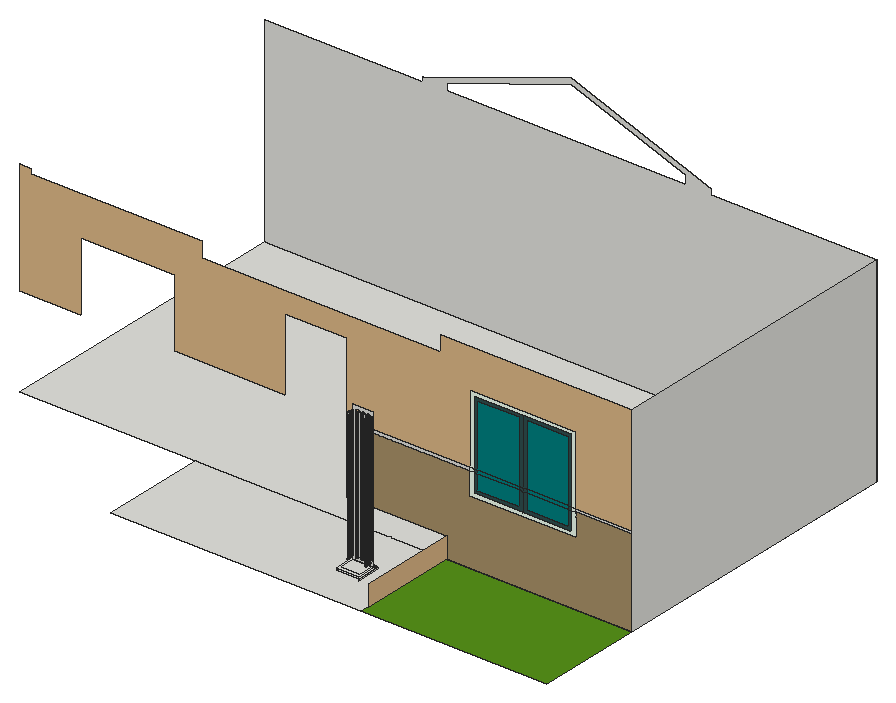
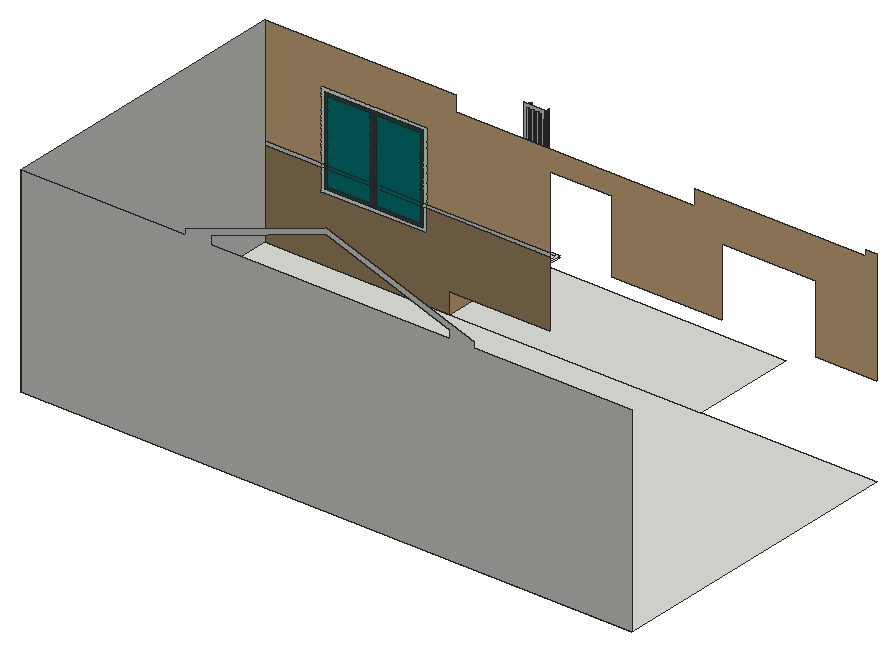
# SketchUp Ruby script. Lengths in inches.
U = 1.inch
M = Sketchup.active_model
def pt(a) = Geom::Point3d.new(a.map { |v| v * U })
def face(e, loops, mat)
  f = e.add_face(loops[0].map { |a| pt(a) })
  loops[1..].each { |l| e.add_face(l.map { |a| pt(a) }).erase! }
  f.material = f.back_material = mat if mat
  f
end
# faces: each face lists its corners as indices into pts; further lists are holes
def faces(e, pts, list, mat = nil) = list.each { |f| face(e, (f[0].is_a?(Array) ? f : [f]).map { |l| l.map { |i| pts[i] } }, mat) }
# xy, xz, yz: faces in a plane at the given z, y or x. An outline is a flat list of corners, or four numbers for a rectangle; further outlines are holes
def ring(l) = l.size == 4 ? [[l[0], l[1]], [l[2], l[1]], [l[2], l[3]], [l[0], l[3]]] : l.each_slice(2).to_a
def flat(e, list, mat, &to3) = list.each { |f| face(e, (f[0].is_a?(Array) ? f : [f]).map { |l| ring(l).map { |u, v| to3.(u, v) } }, mat) }
def xy(e, z, list, mat = nil) = flat(e, list, mat) { |x, y| [x, y, z] }
def xz(e, y, list, mat = nil) = flat(e, list, mat) { |x, z| [x, y, z] }
def yz(e, x, list, mat = nil) = flat(e, list, mat) { |y, z| [x, y, z] }
def lines(e, pts, list) = list.each { |a, b| e.add_line(pt(pts[a]), pt(pts[b])) }
# prism: a flat outline (further loops are holes) pulled along v
def prism(e, loops, v, mat = nil)
  f = face(e, loops, mat); d = Geom::Vector3d.new(v.map { |x| x * U })
  f.pushpull(f.normal.samedirection?(d) ? d.length : -d.length)
end
def box(e, o, s, mat = nil) = prism(e, [[o, [o[0] + s[0], o[1], o[2]], [o[0] + s[0], o[1] + s[1], o[2]], [o[0], o[1] + s[1], o[2]]]], [0, 0, s[2]], mat)
def at(x, y, z, deg = 0) = Geom::Transformation.translation(pt([x, y, z])) * Geom::Transformation.rotation(ORIGIN, Z_AXIS, deg.degrees)
def axes(o, x, y, z) = Geom::Transformation.new([*x, 0, *y, 0, *z, 0, *pt(o).to_a, 1])
def part(name) = M.definitions.add(name)
# library, detail: a bought-in or finely detailed component or shape, given as its bounding box
def library(name, o, s) = part(name).tap { |d| box(d.entities, o, s) }
def detail(e, o, s) = box(e.add_group.entities, o, s)
def put(e, d, t, mat = nil) = e.add_instance(d, t).tap { |i| i.material = mat if mat }
def group(e, t, mat = nil) = e.add_group.tap { |g| g.transformation = t; g.material = mat if mat }.entities
root = M.entities
M.materials.add("[0036_BurlyWood]").color = [222, 184, 135]
M.materials.add("[0066_Honeydew]").color = [240, 255, 240]
M.materials.add("[0078_DarkSlateGray]").color = [47, 79, 79]
M.materials.add("[0079_Teal]").color = [0, 128, 128]
M.materials.add("[Stone Sandstone Ashlar Light]").color = [168, 145, 104]
M.materials.add("[Vegetation Honey Locust]").color = [86, 145, 25]
xy(root,0,[[103.43,1.91,251.04,64.75],[0,64.75,360,244.75]])
xy(root,0,[[251.04,1.91,360,64.75]],"[Vegetation Honey Locust]")
xy(root,12.13,[[231.46,8.1,244.45,21.09]])
xy(root,13.17,[[[231.46,8.1,244.45,21.09],[232.25,9.67,243.67,19.51]]])
xz(root,19.51,[[[232.25,13.17,243.67,94.95],[240.91,14.97,241.17,15,241.4,15.09,241.61,15.24,241.76,15.42,241.86,15.64,241.9,15.875,241.9,92.25,241.86,92.48,241.76,92.7,241.61,92.89,241.4,93.03,241.17,93.12,240.91,93.15,240.66,93.12,240.42,93.03,240.22,92.89,240.06,92.7,239.96,92.48,239.93,92.25,239.93,15.875,239.96,15.64,240.06,15.42,240.22,15.24,240.42,15.09,240.66,15],[235.01,14.97,235.26,15,235.5,15.09,235.7,15.24,235.86,15.42,235.96,15.64,235.99,15.875,235.99,92.25,235.96,92.48,235.86,92.7,235.7,92.89,235.5,93.03,235.26,93.12,235.01,93.15,234.75,93.12,234.51,93.03,234.31,92.89,234.15,92.7,234.05,92.48,234.02,92.25,234.02,15.875,234.05,15.64,234.15,15.42,234.31,15.24,234.51,15.09,234.75,15],[237.96,14.97,238.21,15,238.45,15.09,238.65,15.24,238.8125,15.42,238.91,15.64,238.94,15.875,238.94,92.25,238.91,92.48,238.8125,92.7,238.65,92.89,238.45,93.03,238.21,93.12,237.96,93.15,237.7,93.12,237.47,93.03,237.26,92.89,237.11,92.7,237.01,92.48,236.97,92.25,236.97,15.875,237.01,15.64,237.11,15.42,237.26,15.24,237.47,15.09,237.7,15]]])
xz(root,21.09,[[231.46,12.13,244.45,13.02],[231.46,13.02,244.45,13.17]])
xz(root,21.61,[[230.94,11.46,244.97,12.13]])
xz(root,64.75,[[191.99,51.19,264.92,53.19],[326.96,51.19,360,53.19]])
xz(root,64.75,[[0,53.19,35.4,53.19,35.4,93.75,90.9,93.75,90.9,53.19,155.99,53.19,155.99,96,191.99,96,191.99,53.19,264.92,53.19,264.92,93.75,326.96,93.75,326.96,53.19,360,53.19,360,117,247.8,117,247.8,108.125,106.86,108.125,106.86,117,6.32,117,6.32,120,0,120]],"[0036_BurlyWood]")
xz(root,64.75,[[264.92,38.25,326.96,38.25,326.96,51.19,324.96,51.19,324.96,40.25,266.92,40.25,266.92,51.19,264.92,51.19],[264.92,51.19,266.92,53.19],[324.96,51.19,326.96,53.19],[264.92,53.19,266.92,53.19,266.92,91.75,324.96,91.75,324.96,53.19,326.96,53.19,326.96,93.75,264.92,93.75]],"[0066_Honeydew]")
xz(root,64.75,[[266.92,40.25,295.9375,40.25,295.9375,51.19,293.9375,51.19,293.9375,42.25,268.92,42.25,268.92,51.19,266.92,51.19],[295.9375,40.25,324.96,40.25,324.96,51.19,322.96,51.19,322.96,42.25,297.9375,42.25,297.9375,51.19,295.9375,51.19],[266.92,51.19,268.92,53.19],[293.9375,51.19,295.9375,53.19],[295.9375,51.19,297.9375,53.19],
  [322.96,51.19,324.96,53.19],[266.92,53.19,268.92,53.19,268.92,89.75,293.9375,89.75,293.9375,53.19,295.9375,53.19,295.9375,91.75,266.92,91.75],[295.9375,53.19,297.9375,53.19,297.9375,89.75,322.96,89.75,322.96,53.19,324.96,53.19,324.96,91.75,295.9375,91.75]],"[0078_DarkSlateGray]")
xz(root,64.75,[[268.92,42.25,293.9375,51.19],[297.9375,42.25,322.96,51.19],[268.92,51.19,293.9375,53.19],[297.9375,51.19,322.96,53.19],[268.92,53.19,293.9375,89.75],
  [297.9375,53.19,322.96,89.75]],"[0079_Teal]")
xz(root,64.75,[[251.04,0,360,0,360,51.19,326.96,51.19,326.96,38.25,264.92,38.25,264.92,51.19,191.99,51.19,191.99,12,251.04,12]],"[Stone Sandstone Ashlar Light]")
xz(root,244.75,[[[0,0,0,117,93.16,117,93.16,119.98,93.21,120,180,149.8,262.52,120,262.6,119.97,262.6,117,360,117,360,0],[106.86,117,247.8,117,247.8,122.125,179.96,146.625,106.86,121.52]]])
yz(root,244.97,[[7.58,11.46,21.61,12.13]])
yz(root,251.04,[[7.125,0,64.75,12]],"[0036_BurlyWood]")
yz(root,360,[[64.75,0,244.75,117]])
p = [[231.14,21.41,12.15],[231.2,21.35,12.2],[244.71,21.35,12.2],[244.78,21.41,12.15],[231.11,21.44,12.13],[244.81,21.44,12.13],
  [231.26,21.29,12.27],[244.65,21.29,12.27],[231.32,21.24,12.36],[244.6,21.24,12.36],[231.36,21.1875,12.47],[244.55,21.1875,12.47],
  [231.4,21.15,12.59],[244.52,21.15,12.59],[231.43,21.12,12.73],[244.49,21.12,12.73],[231.45,21.1,12.87],[244.47,21.1,12.87],
  [231.46,21.09,13.02],[244.45,21.09,13.02],[234.88,19.29,15],[234.76,19.09,15.09],[234.88,19.04,15.09],[234.94,19.27,15],
  [235.01,19.02,15.09],[235.01,19.26,15],[235.13,19.04,15.09],[235.07,19.27,15],[235.25,19.09,15.09],[235.13,19.29,15],
  [237.83,19.29,15],[237.71,19.09,15.09],[237.83,19.04,15.09],[237.89,19.27,15],[237.96,19.02,15.09],[237.96,19.26,15],
  [238.09,19.04,15.09],[238.02,19.27,15],[238.2,19.09,15.09],[238.09,19.29,15],[240.78,19.29,15],[240.67,19.09,15.09],
  [240.78,19.04,15.09],[240.85,19.27,15],[240.91,19.02,15.09],[240.91,19.26,15],[241.04,19.04,15.09],[240.98,19.27,15],
  [241.16,19.09,15.09],[241.04,19.29,15],[234.83,19.33,15],[234.66,19.17,15.09],[235.35,19.17,15.09],[235.1875,19.33,15],
  [237.78,19.33,15],[237.61,19.17,15.09],[238.31,19.17,15.09],[238.14,19.33,15],[240.73,19.33,15],[240.5625,19.17,15.09],
  [241.26,19.17,15.09],[241.09,19.33,15],[234.78,19.39,15],[234.58,19.27,15.09],[235.43,19.27,15.09],[235.23,19.39,15],
  [237.74,19.39,15],[237.53,19.27,15.09],[238.38,19.27,15.09],[238.18,19.39,15],[240.69,19.39,15],[240.48,19.27,15.09],
  [241.34,19.27,15.09],[241.13,19.39,15],[234.76,19.45,15],[234.53,19.39,15.09],[235.01,19.51,14.97],[235.48,19.39,15.09],
  [235.25,19.45,15],[237.71,19.45,15],[237.48,19.39,15.09],[237.96,19.51,14.97],[238.43,19.39,15.09],[238.2,19.45,15],
  [240.67,19.45,15],[240.4375,19.39,15.09],[240.91,19.51,14.97],[241.39,19.39,15.09],[241.16,19.45,15],[234.75,19.51,15],
  [234.51,19.51,15.09],[235.26,19.51,15],[235.5,19.51,15.09],[237.7,19.51,15],[237.47,19.51,15.09],[238.21,19.51,15],
  [238.45,19.51,15.09],[240.66,19.51,15],[240.42,19.51,15.09],[241.17,19.51,15],[241.4,19.51,15.09],[234.66,18.91,15.24],
  [234.83,18.84,15.24],[235.01,18.82,15.24],[235.1875,18.84,15.24],[235.35,18.91,15.24],[237.61,18.91,15.24],[237.78,18.84,15.24],
  [237.96,18.82,15.24],[238.14,18.84,15.24],[238.31,18.91,15.24],[240.5625,18.91,15.24],[240.73,18.84,15.24],[240.91,18.82,15.24],
  [241.09,18.84,15.24],[241.26,18.91,15.24],[234.51,19.02,15.24],[235.5,19.02,15.24],[237.47,19.02,15.24],[238.45,19.02,15.24],
  [240.42,19.02,15.24],[241.4,19.02,15.24],[234.4,19.17,15.24],[235.61,19.17,15.24],[237.36,19.17,15.24],[238.5625,19.17,15.24],
  [240.31,19.17,15.24],[241.51,19.17,15.24],[234.33,19.33,15.24],[235.68,19.33,15.24],[237.29,19.33,15.24],[238.63,19.33,15.24],
  [240.24,19.33,15.24],[241.58,19.33,15.24],[234.31,19.51,15.24],[235.7,19.51,15.24],[237.26,19.51,15.24],[238.65,19.51,15.24],
  [240.22,19.51,15.24],[241.61,19.51,15.24],[232.25,14.59,15.23],[232.5,14.59,15.27],[232.5,14.66,15.27],[232.47,14.72,15.27],
  [232.43,14.77,15.27],[232.38,14.8125,15.27],[232.32,14.84,15.27],[232.25,14.85,15.27],[243.41,14.59,15.27],[243.67,14.59,15.23],
  [243.42,14.66,15.27],[243.45,14.72,15.27],[243.49,14.77,15.27],[243.54,14.8125,15.27],[243.6,14.84,15.27],[243.67,14.85,15.27],
  [232.25,17.29,15.27],[232.32,17.3,15.27],[232.25,17.55,15.23],[232.38,17.32,15.27],[232.43,17.37,15.27],[243.67,17.55,15.23],
  [243.54,17.32,15.27],[243.6,17.3,15.27],[243.49,17.37,15.27],[243.67,17.29,15.27],[232.47,17.42,15.27],[232.5,17.48,15.27],
  [243.45,17.42,15.27],[243.42,17.48,15.27],[232.5,17.55,15.27],[232.5,17.61,15.27],[232.47,17.67,15.27],[232.43,17.73,15.27],
  [232.38,17.77,15.27],[232.32,17.79,15.27],[232.25,17.8,15.27],[243.41,17.55,15.27],[243.42,17.61,15.27],[243.45,17.67,15.27],
  [243.49,17.73,15.27],[243.54,17.77,15.27],[243.6,17.79,15.27],[243.67,17.8,15.27],[234.58,18.78,15.42],[234.78,18.69,15.42],
  [235.01,18.66,15.42],[235.23,18.69,15.42],[235.43,18.78,15.42],[237.53,18.78,15.42],[237.74,18.69,15.42],[237.96,18.66,15.42],
  [238.18,18.69,15.42],[238.38,18.78,15.42],[240.48,18.78,15.42],[240.69,18.69,15.42],[240.91,18.66,15.42],[241.13,18.69,15.42],
  [241.34,18.78,15.42],[234.4,18.91,15.42],[235.61,18.91,15.42],[237.36,18.91,15.42],[238.5625,18.91,15.42],[240.31,18.91,15.42],
  [241.51,18.91,15.42],[234.27,19.09,15.42],[235.74,19.09,15.42],[237.22,19.09,15.42],[238.7,19.09,15.42],[240.17,19.09,15.42],
  [241.65,19.09,15.42],[234.18,19.29,15.42],[235.83,19.29,15.42],[237.14,19.29,15.42],[238.78,19.29,15.42],[240.09,19.29,15.42],
  [241.73,19.29,15.42],[234.15,19.51,15.42],[235.86,19.51,15.42],[237.11,19.51,15.42],[238.8125,19.51,15.42],[240.06,19.51,15.42],
  [241.76,19.51,15.42],[232.74,14.59,15.36],[232.73,14.72,15.36],[243.17,14.59,15.36],[243.19,14.72,15.36],[232.68,14.84,15.36],
  [232.6,14.94,15.36],[243.24,14.84,15.36],[243.32,14.94,15.36],[232.38,15.07,15.36],[232.25,15.08,15.36],[232.5,15.02,15.36],
  [243.42,15.02,15.36],[243.54,15.07,15.36],[243.67,15.08,15.36],[232.25,17.05,15.36],[232.38,17.07,15.36],[232.5,17.12,15.36],
  [232.6,17.2,15.36],[243.32,17.2,15.36],[243.42,17.12,15.36],[243.54,17.07,15.36],[243.67,17.05,15.36],[232.68,17.3,15.36],
  [243.24,17.3,15.36],[232.73,17.42,15.36],[243.19,17.42,15.36],[232.74,17.55,15.36],[243.17,17.55,15.36],[232.73,17.67,15.36],
  [243.19,17.67,15.36],[232.68,17.79,15.36],[243.24,17.79,15.36],[232.6,17.89,15.36],[232.5,17.97,15.36],[243.32,17.89,15.36],
  [243.42,17.97,15.36],[232.38,18.02,15.36],[232.25,18.04,15.36],[243.54,18.02,15.36],[243.67,18.04,15.36],[232.95,14.59,15.5],
  [232.92,14.77,15.5],[242.97,14.59,15.5],[242.99,14.77,15.5],[232.85,14.94,15.5],[243.0625,14.94,15.5],[232.74,15.08,15.5],
  [243.17,15.08,15.5],[232.6,15.2,15.5],[243.32,15.2,15.5],[232.43,15.26,15.5],[243.49,15.26,15.5],[232.25,15.29,15.5],
  [243.67,15.29,15.5],[232.25,16.85,15.5],[232.43,16.875,15.5],[243.49,16.875,15.5],[243.67,16.85,15.5],[232.6,16.94,15.5],
  [232.74,17.05,15.5],[243.17,17.05,15.5],[243.32,16.94,15.5],[232.85,17.2,15.5],[243.0625,17.2,15.5],[232.92,17.37,15.5],
  [242.99,17.37,15.5],[232.95,17.55,15.5],[242.97,17.55,15.5],[232.92,17.73,15.5],[242.99,17.73,15.5],[232.85,17.89,15.5],
  [243.0625,17.89,15.5],[232.74,18.04,15.5],[243.17,18.04,15.5],[232.6,18.15,15.5],[243.32,18.15,15.5],[232.43,18.22,15.5],
  [232.25,18.24,15.5],[243.49,18.22,15.5],[243.67,18.24,15.5],[234.53,18.69,15.64],[234.76,18.6,15.64],[235.01,18.5625,15.64],
  [235.25,18.6,15.64],[235.48,18.69,15.64],[237.48,18.69,15.64],[237.71,18.6,15.64],[237.96,18.5625,15.64],[238.2,18.6,15.64],
  [238.43,18.69,15.64],[240.4375,18.69,15.64],[240.67,18.6,15.64],[240.91,18.5625,15.64],[241.16,18.6,15.64],[241.39,18.69,15.64],
  [234.33,18.84,15.64],[235.68,18.84,15.64],[237.29,18.84,15.64],[238.63,18.84,15.64],[240.24,18.84,15.64],[241.58,18.84,15.64],
  [234.18,19.04,15.64],[235.83,19.04,15.64],[237.14,19.04,15.64],[238.78,19.04,15.64],[240.09,19.04,15.64],[241.73,19.04,15.64],
  [234.09,19.27,15.64],[235.92,19.27,15.64],[237.04,19.27,15.64],[238.875,19.27,15.64],[239.99,19.27,15.64],[241.83,19.27,15.64],
  [234.05,19.51,15.64],[235.96,19.51,15.64],[237.01,19.51,15.64],[238.91,19.51,15.64],[239.96,19.51,15.64],[241.86,19.51,15.64],
  [233.1,14.59,15.69],[233.07,14.8125,15.69],[242.81,14.59,15.69],[242.84,14.8125,15.69],[232.99,15.02,15.69],[242.93,15.02,15.69],
  [232.85,15.2,15.69],[243.0625,15.2,15.69],[232.68,15.33,15.69],[243.24,15.33,15.69],[232.47,15.42,15.69],[243.45,15.42,15.69],
  [232.25,15.44,15.69],[243.67,15.44,15.69],[232.25,16.69,15.69],[232.47,16.72,15.69],[232.68,16.81,15.69],[243.24,16.81,15.69],
  [243.45,16.72,15.69],[243.67,16.69,15.69],[232.85,16.94,15.69],[243.0625,16.94,15.69],[232.99,17.12,15.69],[242.93,17.12,15.69],
  [233.07,17.32,15.69],[242.84,17.32,15.69],[233.1,17.55,15.69],[242.81,17.55,15.69],[233.07,17.77,15.69],[242.84,17.77,15.69],
  [232.99,17.97,15.69],[242.93,17.97,15.69],[232.85,18.15,15.69],[243.0625,18.15,15.69],[232.68,18.28,15.69],[243.24,18.28,15.69],
  [232.47,18.37,15.69],[243.45,18.37,15.69],[232.25,18.4,15.69],[243.67,18.4,15.69],[234.75,18.5625,15.875],[235.01,18.53,15.875],
  [235.26,18.5625,15.875],[237.7,18.5625,15.875],[237.96,18.53,15.875],[238.21,18.5625,15.875],[240.66,18.5625,15.875],[240.91,18.53,15.875],
  [241.17,18.5625,15.875],[234.51,18.66,15.875],[235.5,18.66,15.875],[237.47,18.66,15.875],[238.45,18.66,15.875],[240.42,18.66,15.875],
  [241.4,18.66,15.875],[234.31,18.82,15.875],[235.7,18.82,15.875],[237.26,18.82,15.875],[238.65,18.82,15.875],[240.22,18.82,15.875],
  [241.61,18.82,15.875],[234.15,19.02,15.875],[235.86,19.02,15.875],[237.11,19.02,15.875],[238.8125,19.02,15.875],[240.06,19.02,15.875],
  [241.76,19.02,15.875],[234.05,19.26,15.875],[235.96,19.26,15.875],[237.01,19.26,15.875],[238.91,19.26,15.875],[239.96,19.26,15.875],
  [241.86,19.26,15.875],[234.02,19.51,15.875],[235.99,19.51,15.875],[236.97,19.51,15.875],[238.94,19.51,15.875],[239.93,19.51,15.875],
  [241.9,19.51,15.875],[233.2,14.59,15.9],[233.17,14.84,15.9],[242.72,14.59,15.9],[242.75,14.84,15.9],[233.07,15.07,15.9],
  [242.84,15.07,15.9],[232.92,15.26,15.9],[242.99,15.26,15.9],[232.73,15.42,15.9],[243.19,15.42,15.9],[232.5,15.51,15.9],
  [243.42,15.51,15.9],[232.25,15.54,15.9],[243.67,15.54,15.9],[232.25,16.59,15.9],[232.5,16.625,15.9],[232.73,16.72,15.9],
  [243.19,16.72,15.9],[243.42,16.625,15.9],[243.67,16.59,15.9],[232.92,16.875,15.9],[242.99,16.875,15.9],[233.07,17.07,15.9],
  [242.84,17.07,15.9],[233.17,17.3,15.9],[242.75,17.3,15.9],[233.2,17.55,15.9],[242.72,17.55,15.9],[233.17,17.79,15.9],
  [242.75,17.79,15.9],[233.07,18.02,15.9],[242.84,18.02,15.9],[232.92,18.22,15.9],[242.99,18.22,15.9],[232.73,18.37,15.9],
  [243.19,18.37,15.9],[232.5,18.46,15.9],[243.42,18.46,15.9],[232.25,18.5,15.9],[243.67,18.5,15.9],[233.23,14.59,16.14],
  [233.2,14.85,16.14],[242.68,14.59,16.14],[242.72,14.85,16.14],[233.1,15.08,16.14],[242.81,15.08,16.14],[232.95,15.29,16.14],
  [242.97,15.29,16.14],[232.74,15.44,16.14],[243.17,15.44,16.14],[232.5,15.54,16.14],[243.41,15.54,16.14],[232.25,15.58,16.14],
  [243.67,15.58,16.14],[232.25,16.5625,16.14],[232.5,16.59,16.14],[232.74,16.69,16.14],[243.17,16.69,16.14],[243.41,16.59,16.14],
  [243.67,16.5625,16.14],[232.95,16.85,16.14],[242.97,16.85,16.14],[233.1,17.05,16.14],[242.81,17.05,16.14],[233.2,17.29,16.14],
  [242.72,17.29,16.14],[233.23,17.55,16.14],[242.68,17.55,16.14],[233.2,17.8,16.14],[242.72,17.8,16.14],[233.1,18.04,16.14],
  [242.81,18.04,16.14],[232.95,18.24,16.14],[242.97,18.24,16.14],[232.74,18.4,16.14],[243.17,18.4,16.14],[232.5,18.5,16.14],
  [243.41,18.5,16.14],[232.25,18.53,16.14],[234.75,18.5625,92.25],[235.01,18.53,92.25],[235.26,18.5625,92.25],[237.7,18.5625,92.25],
  [237.96,18.53,92.25],[238.21,18.5625,92.25],[240.66,18.5625,92.25],[240.91,18.53,92.25],[241.17,18.5625,92.25],[243.67,18.53,16.14],
  [234.51,18.66,92.25],[235.5,18.66,92.25],[237.47,18.66,92.25],[238.45,18.66,92.25],[240.42,18.66,92.25],[241.4,18.66,92.25],
  [234.31,18.82,92.25],[235.7,18.82,92.25],[237.26,18.82,92.25],[238.65,18.82,92.25],[240.22,18.82,92.25],[241.61,18.82,92.25],
  [234.15,19.02,92.25],[235.86,19.02,92.25],[237.11,19.02,92.25],[238.8125,19.02,92.25],[240.06,19.02,92.25],[241.76,19.02,92.25],
  [234.05,19.26,92.25],[235.96,19.26,92.25],[237.01,19.26,92.25],[238.91,19.26,92.25],[239.96,19.26,92.25],[241.86,19.26,92.25],
  [234.02,19.51,92.25],[235.99,19.51,92.25],[236.97,19.51,92.25],[238.94,19.51,92.25],[239.93,19.51,92.25],[241.9,19.51,92.25],
  [233.23,14.59,92.51],[233.2,14.85,92.51],[242.72,14.85,92.51],[242.68,14.59,92.51],[233.1,15.08,92.51],[242.81,15.08,92.51],
  [232.95,15.29,92.51],[242.97,15.29,92.51],[232.74,15.44,92.51],[243.17,15.44,92.51],[232.5,15.54,92.51],[243.41,15.54,92.51],
  [232.25,15.58,92.51],[243.67,15.58,92.51],[232.25,16.5625,92.51],[232.5,16.59,92.51],[232.74,16.69,92.51],[243.17,16.69,92.51],
  [243.41,16.59,92.51],[243.67,16.5625,92.51],[232.95,16.85,92.51],[242.97,16.85,92.51],[233.1,17.05,92.51],[242.81,17.05,92.51],
  [233.2,17.29,92.51],[242.72,17.29,92.51],[233.23,17.55,92.51],[242.68,17.55,92.51],[233.2,17.8,92.51],[242.72,17.8,92.51],
  [233.1,18.04,92.51],[242.81,18.04,92.51],[232.95,18.24,92.51],[242.97,18.24,92.51],[232.74,18.4,92.51],[243.17,18.4,92.51],
  [232.5,18.5,92.51],[243.41,18.5,92.51],[232.25,18.53,92.51],[243.67,18.53,92.51]]
faces(root,p,[[0,1,2,3],[4,0,3,5],[1,6,7,2],[6,8,9,7],[8,10,11,9],[10,12,13,11],[12,14,15,13],[14,16,17,15],
  [16,18,19,17],[20,21,22,23],[23,22,24,25],[25,24,26,27],[27,26,28,29],[30,31,32,33],[33,32,34,35],[35,34,36,37],
  [37,36,38,39],[40,41,42,43],[43,42,44,45],[45,44,46,47],[47,46,48,49],[50,51,21,20],[29,28,52,53],[54,55,31,30],
  [39,38,56,57],[58,59,41,40],[49,48,60,61],[62,63,51,50],[53,52,64,65],[66,67,55,54],[57,56,68,69],[70,71,59,58],
  [61,60,72,73],[74,75,63,62],[76,50,20],[76,62,50],[76,23,25],[76,20,23],[76,25,27],[76,27,29],
  [76,29,53],[76,53,65],[65,64,77,78],[79,80,67,66],[81,66,54],[81,30,33],[81,54,30],[81,33,35],
  [81,35,37],[81,37,39],[81,39,57],[81,57,69],[69,68,82,83],[84,85,71,70],[86,58,40],[86,70,58],
  [86,43,45],[86,40,43],[86,45,47],[86,47,49],[86,49,61],[86,61,73],[73,72,87,88],[74,89,90,75],
  [76,74,62],[74,76,89],[76,65,78],[78,91,76],[77,92,91,78],[79,93,94,80],[81,79,66],[79,81,93],
  [81,69,83],[83,95,81],[82,96,95,83],[84,97,98,85],[86,84,70],[84,86,97],[86,73,88],[88,99,86],
  [87,100,99,88],[21,101,102,22],[22,102,103,24],[24,103,104,26],[26,104,105,28],[31,106,107,32],[32,107,108,34],[34,108,109,36],
  [36,109,110,38],[41,111,112,42],[42,112,113,44],[44,113,114,46],[46,114,115,48],[51,116,101,21],[28,105,117,52],[55,118,106,31],
  [38,110,119,56],[59,120,111,41],[48,115,121,60],[63,122,116,51],[52,117,123,64],[67,124,118,55],[56,119,125,68],[71,126,120,59],
  [60,121,127,72],[75,128,122,63],[64,123,129,77],[80,130,124,67],[68,125,131,82],[85,132,126,71],[72,127,133,87],[75,90,134,128],
  [129,135,92,77],[80,94,136,130],[131,137,96,82],[85,98,138,132],[133,139,100,87],[140,141,142],[140,142,143],[140,143,144],
  [140,144,145],[140,145,146],[146,147,140],[148,149,150],[150,149,151],[151,149,152],[152,149,153],[153,149,154],
  [155,154,149],[156,157,158],[159,158,157],[160,158,159],[161,162,163],[161,164,162],[163,165,161],[166,158,160],
  [167,158,166],[161,168,164],[161,169,168],[170,158,167],[171,158,170],[172,158,171],[173,158,172],[174,158,173],
  [175,158,174],[158,175,176],[161,177,169],[161,178,177],[161,179,178],[161,180,179],[161,181,180],[161,182,181],
  [182,161,183],[101,184,185,102],[102,185,186,103],[103,186,187,104],[104,187,188,105],[106,189,190,107],[107,190,191,108],[108,191,192,109],
  [109,192,193,110],[111,194,195,112],[112,195,196,113],[113,196,197,114],[114,197,198,115],[116,199,184,101],[105,188,200,117],[118,201,189,106],
  [110,193,202,119],[120,203,194,111],[115,198,204,121],[122,205,199,116],[117,200,206,123],[124,207,201,118],[119,202,208,125],[126,209,203,120],
  [121,204,210,127],[128,211,205,122],[123,206,212,129],[130,213,207,124],[125,208,214,131],[132,215,209,126],[127,210,216,133],[128,134,217,211],
  [212,218,135,129],[130,136,219,213],[214,220,137,131],[132,138,221,215],[216,222,139,133],[141,223,224,142],[225,148,150,226],[143,227,228,144],
  [142,224,227,143],[226,150,151,229],[229,151,152,230],[231,232,147,146],[145,233,231,146],[144,228,233,145],[230,152,153,234],[234,153,154,235],
  [236,235,154,155],[237,238,157,156],[239,159,157,238],[240,160,159,239],[164,241,242,162],[162,242,243,163],[243,244,165,163],[245,166,160,240],
  [168,246,241,164],[247,167,166,245],[169,248,246,168],[249,170,167,247],[177,250,248,169],[251,171,170,249],[178,252,250,177],[253,172,171,251],
  [179,254,252,178],[255,173,172,253],[256,174,173,255],[180,257,254,179],[181,258,257,180],[176,175,259,260],[259,175,174,256],[182,261,258,181],
  [182,183,262,261],[223,263,264,224],[265,225,226,266],[224,264,267,227],[266,226,229,268],[227,267,269,228],[268,229,230,270],[228,269,271,233],
  [270,230,234,272],[233,271,273,231],[272,234,235,274],[273,275,232,231],[276,274,235,236],[277,278,238,237],[279,280,244,243],[281,239,238,278],
  [282,240,239,281],[241,283,284,242],[242,284,279,243],[285,245,240,282],[246,286,283,241],[287,247,245,285],[248,288,286,246],[289,249,247,287],
  [250,290,288,248],[291,251,249,289],[252,292,290,250],[293,253,251,291],[254,294,292,252],[295,255,253,293],[257,296,294,254],[297,256,255,295],
  [258,298,296,257],[260,259,299,300],[299,259,256,297],[261,301,298,258],[261,262,302,301],[184,303,304,185],[185,304,305,186],[186,305,306,187],
  [187,306,307,188],[189,308,309,190],[190,309,310,191],[191,310,311,192],[192,311,312,193],[194,313,314,195],[195,314,315,196],[196,315,316,197],
  [197,316,317,198],[199,318,303,184],[188,307,319,200],[201,320,308,189],[193,312,321,202],[203,322,313,194],[198,317,323,204],[205,324,318,199],
  [200,319,325,206],[207,326,320,201],[202,321,327,208],[209,328,322,203],[204,323,329,210],[211,330,324,205],[206,325,331,212],[213,332,326,207],
  [208,327,333,214],[215,334,328,209],[210,329,335,216],[211,217,336,330],[331,337,218,212],[213,219,338,332],[333,339,220,214],[215,221,340,334],
  [335,341,222,216],[263,342,343,264],[344,265,266,345],[264,343,346,267],[345,266,268,347],[267,346,348,269],[347,268,270,349],[269,348,350,271],
  [349,270,272,351],[271,350,352,273],[351,272,274,353],[352,354,275,273],[355,353,274,276],[356,357,278,277],[358,281,278,357],[284,359,360,279],
  [360,361,280,279],[362,282,281,358],[283,363,359,284],[364,285,282,362],[286,365,363,283],[366,287,285,364],[288,367,365,286],[368,289,287,366],
  [290,369,367,288],[370,291,289,368],[292,371,369,290],[372,293,291,370],[294,373,371,292],[374,295,293,372],[296,375,373,294],[376,297,295,374],
  [298,377,375,296],[378,299,297,376],[301,379,377,298],[300,299,378,380],[301,302,381,379],[304,382,383,305],[305,383,384,306],[309,385,386,310],
  [310,386,387,311],[314,388,389,315],[315,389,390,316],[303,391,382,304],[306,384,392,307],[308,393,385,309],[311,387,394,312],[313,395,388,314],
  [316,390,396,317],[318,397,391,303],[307,392,398,319],[320,399,393,308],[312,394,400,321],[322,401,395,313],[317,396,402,323],[324,403,397,318],
  [319,398,404,325],[326,405,399,320],[321,400,406,327],[328,407,401,322],[323,402,408,329],[330,409,403,324],[325,404,410,331],[332,411,405,326],
  [327,406,412,333],[334,413,407,328],[329,408,414,335],[330,336,415,409],[410,416,337,331],[332,338,417,411],[412,418,339,333],[334,340,419,413],
  [414,420,341,335],[342,421,422,343],[423,344,345,424],[343,422,425,346],[424,345,347,426],[346,425,427,348],[426,347,349,428],[348,427,429,350],
  [428,349,351,430],[350,429,431,352],[430,351,353,432],[431,433,354,352],[434,432,353,355],[435,436,357,356],[437,358,357,436],[359,438,439,360],
  [439,440,361,360],[441,362,358,437],[363,442,438,359],[443,364,362,441],[365,444,442,363],[445,366,364,443],[367,446,444,365],[447,368,366,445],
  [369,448,446,367],[449,370,368,447],[371,450,448,369],[451,372,370,449],[373,452,450,371],[453,374,372,451],[375,454,452,373],[455,376,374,453],
  [377,456,454,375],[457,378,376,455],[379,458,456,377],[380,378,457,459],[379,381,460,458],[421,461,462,422],[463,423,424,464],[422,462,465,425],
  [464,424,426,466],[425,465,467,427],[466,426,428,468],[427,467,469,429],[468,428,430,470],[429,469,471,431],[470,430,432,472],[471,473,433,431],
  [474,472,432,434],[475,476,436,435],[477,437,436,476],[438,478,479,439],[479,480,440,439],[481,441,437,477],[442,482,478,438],[483,443,441,481],
  [444,484,482,442],[485,445,443,483],[446,486,484,444],[487,447,445,485],[448,488,486,446],[489,449,447,487],[450,490,488,448],[491,451,449,489],
  [452,492,490,450],[493,453,451,491],[454,494,492,452],[495,455,453,493],[456,496,494,454],[497,457,455,495],[458,498,496,456],[459,457,497,499],
  [383,382,500,501],[384,383,501,502],[386,385,503,504],[387,386,504,505],[389,388,506,507],[390,389,507,508],[458,460,509,498],[382,391,510,500],
  [392,384,502,511],[385,393,512,503],[394,387,505,513],[388,395,514,506],[396,390,508,515],[391,397,516,510],[398,392,511,517],[393,399,518,512],
  [400,394,513,519],[395,401,520,514],[402,396,515,521],[397,403,522,516],[404,398,517,523],[399,405,524,518],[406,400,519,525],[401,407,526,520],
  [408,402,521,527],[403,409,528,522],[410,404,523,529],[405,411,530,524],[412,406,525,531],[407,413,532,526],[414,408,527,533],[409,415,534,528],
  [416,410,529,535],[411,417,536,530],[418,412,531,537],[413,419,538,532],[420,414,533,539],[462,461,540,541],[463,464,542,543],[465,462,541,544],
  [464,466,545,542],[467,465,544,546],[466,468,547,545],[469,467,546,548],[468,470,549,547],[471,469,548,550],[470,472,551,549],[473,471,550,552],
  [472,474,553,551],[476,475,554,555],[477,476,555,556],[479,478,557,558],[480,479,558,559],[481,477,556,560],[478,482,561,557],[483,481,560,562],
  [482,484,563,561],[485,483,562,564],[484,486,565,563],[487,485,564,566],[486,488,567,565],[489,487,566,568],[488,490,569,567],[491,489,568,570],
  [490,492,571,569],[493,491,570,572],[492,494,573,571],[495,493,572,574],[494,496,575,573],[497,495,574,576],[496,498,577,575],[499,497,576,578],
  [498,509,579,577]])
